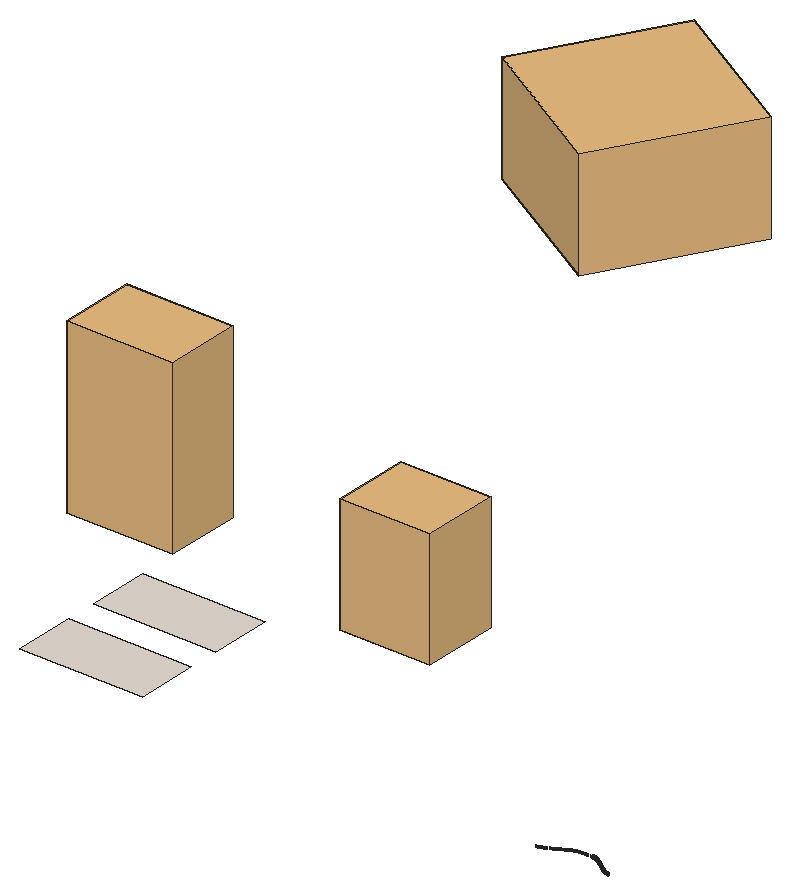
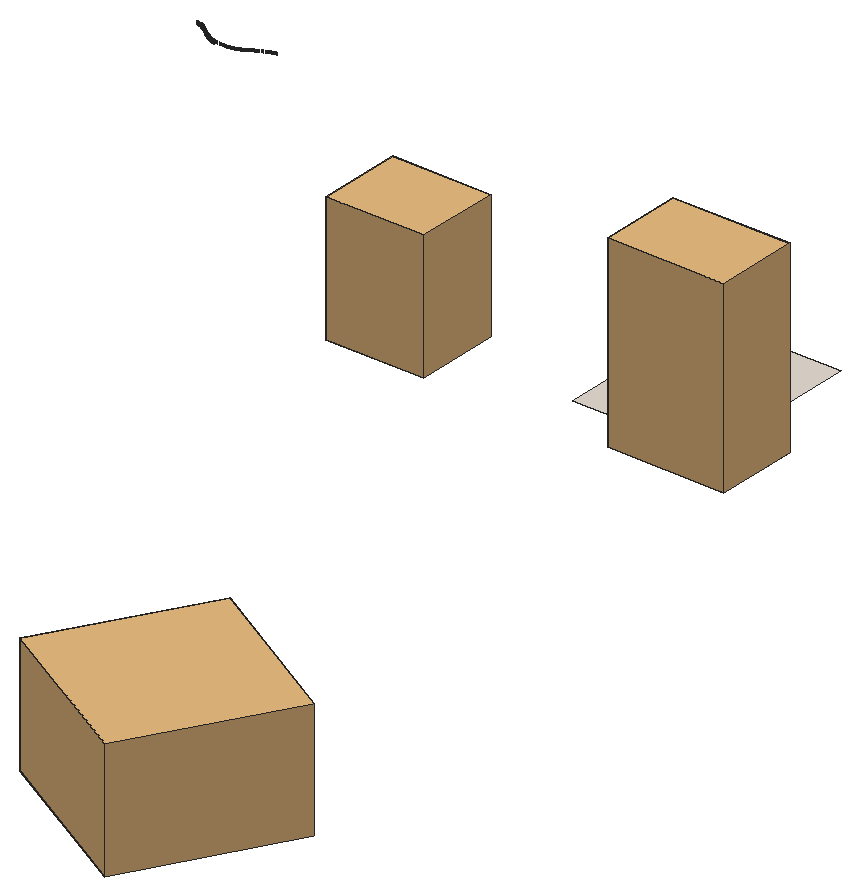
# SketchUp Ruby script. Lengths in inches.
U = 1.inch
M = Sketchup.active_model
def pt(a) = Geom::Point3d.new(a.map { |v| v * U })
def face(e, loops, mat)
  f = e.add_face(loops[0].map { |a| pt(a) })
  loops[1..].each { |l| e.add_face(l.map { |a| pt(a) }).erase! }
  f.material = f.back_material = mat if mat
  f
end
# faces: each face lists its corners as indices into pts; further lists are holes
def faces(e, pts, list, mat = nil) = list.each { |f| face(e, (f[0].is_a?(Array) ? f : [f]).map { |l| l.map { |i| pts[i] } }, mat) }
# xy, xz, yz: faces in a plane at the given z, y or x. An outline is a flat list of corners, or four numbers for a rectangle; further outlines are holes
def ring(l) = l.size == 4 ? [[l[0], l[1]], [l[2], l[1]], [l[2], l[3]], [l[0], l[3]]] : l.each_slice(2).to_a
def flat(e, list, mat, &to3) = list.each { |f| face(e, (f[0].is_a?(Array) ? f : [f]).map { |l| ring(l).map { |u, v| to3.(u, v) } }, mat) }
def xy(e, z, list, mat = nil) = flat(e, list, mat) { |x, y| [x, y, z] }
def xz(e, y, list, mat = nil) = flat(e, list, mat) { |x, z| [x, y, z] }
def yz(e, x, list, mat = nil) = flat(e, list, mat) { |y, z| [x, y, z] }
def lines(e, pts, list) = list.each { |a, b| e.add_line(pt(pts[a]), pt(pts[b])) }
# prism: a flat outline (further loops are holes) pulled along v
def prism(e, loops, v, mat = nil)
  f = face(e, loops, mat); d = Geom::Vector3d.new(v.map { |x| x * U })
  f.pushpull(f.normal.samedirection?(d) ? d.length : -d.length)
end
def box(e, o, s, mat = nil) = prism(e, [[o, [o[0] + s[0], o[1], o[2]], [o[0] + s[0], o[1] + s[1], o[2]], [o[0], o[1] + s[1], o[2]]]], [0, 0, s[2]], mat)
def at(x, y, z, deg = 0) = Geom::Transformation.translation(pt([x, y, z])) * Geom::Transformation.rotation(ORIGIN, Z_AXIS, deg.degrees)
def axes(o, x, y, z) = Geom::Transformation.new([*x, 0, *y, 0, *z, 0, *pt(o).to_a, 1])
def part(name) = M.definitions.add(name)
# library, detail: a bought-in or finely detailed component or shape, given as its bounding box
def library(name, o, s) = part(name).tap { |d| box(d.entities, o, s) }
def detail(e, o, s) = box(e.add_group.entities, o, s)
def put(e, d, t, mat = nil) = e.add_instance(d, t).tap { |i| i.material = mat if mat }
def group(e, t, mat = nil) = e.add_group.tap { |g| g.transformation = t; g.material = mat if mat }.entities
root = M.entities
M.materials.add("Marble_01_1K").color = [230, 221, 211]
M.materials.add("Marble_07_1K").color = [36, 34, 36]
c1 = library("Group\#26",[0,0,0],[90.2,76.39,117.66])
c2 = library("Group\#20",[0,0,0],[118.64,83.7,191])
c3 = library("Group\#158",[-18.75,-2.45,9.86],[64.9,62.99,42.73])
xy(root,2,[[111.43,816.64,159.43,840.64],[111.43,852.64,159.43,876.64]],"Marble_01_1K")
xz(root,802.19,[[347.97,18,348,19]],"Marble_07_1K")
xz(root,802.24,[[347.74,18,347.78,19]],"Marble_07_1K")
xz(root,802.27,[[347.58,18,347.62,19]],"Marble_07_1K")
p = [[358.82,796.23,18],[358.7,796.26,18],[358.7,796.26,19],[358.82,796.23,19],[358.47,796.33,18],[358.36,796.36,18],
  [358.36,796.36,19],[358.47,796.33,19],[358.59,796.29,18],[358.59,796.29,19],[358.13,796.4375,18],[358.01,796.48,18],
  [358.01,796.48,19],[358.13,796.4375,19],[358.24,796.4,18],[358.24,796.4,19],[357.9,796.52,18],[357.79,796.5625,18],
  [357.79,796.5625,19],[357.9,796.52,19],[357.5625,796.65,18],[357.45,796.69,18],[357.45,796.69,19],[357.5625,796.65,19],
  [357.68,796.6,18],[357.68,796.6,19],[357.34,796.74,18],[357.23,796.79,18],[357.23,796.79,19],[357.34,796.74,19],
  [357.12,796.84,18],[357.01,796.89,18],[357.01,796.89,19],[357.12,796.84,19],[356.9,796.9375,18],[356.79,796.99,18],
  [356.79,796.99,19],[356.9,796.9375,19],[356.68,797.04,18],[356.58,797.1,18],[356.58,797.1,19],[356.68,797.04,19],
  [356.47,797.15,18],[356.47,797.15,19],[356.36,797.21,18],[356.26,797.27,18],[356.26,797.27,19],[356.36,797.21,19],
  [356.15,797.32,18],[356.05,797.38,18],[356.05,797.38,19],[356.15,797.32,19],[355.94,797.44,18],[355.84,797.51,18],
  [355.84,797.51,19],[355.94,797.44,19],[355.74,797.57,18],[355.74,797.57,19],[355.64,797.63,18],[355.53,797.7,18],
  [355.53,797.7,19],[355.64,797.63,19],[355.43,797.76,18],[355.43,797.76,19],[355.33,797.83,18],[355.23,797.9,18],
  [355.23,797.9,19],[355.33,797.83,19],[355.13,797.97,18],[355.13,797.97,19],[355.04,798.04,18],[354.9375,798.11,18],
  [354.9375,798.11,19],[355.04,798.04,19],[354.84,798.18,18],[354.84,798.18,19],[354.74,798.25,18],[354.74,798.25,19],
  [354.65,798.33,18],[354.65,798.33,19],[354.55,798.4,18],[354.55,798.4,19],[354.46,798.47,18],[354.46,798.47,19],
  [354.375,798.54,18],[354.29,798.61,18],[354.29,798.61,19],[354.375,798.54,19],[354.2,798.68,18],[354.2,798.68,19],
  [354.11,798.75,18],[354.11,798.75,19],[354.02,798.82,18],[353.93,798.9,18],[353.93,798.9,19],[354.02,798.82,19],
  [353.82,798.99,18],[353.82,798.99,19],[353.71,799.08,18],[353.71,799.08,19],[353.57,799.19,18],[353.57,799.19,19],
  [353.42,799.3,18],[353.42,799.3,19],[353.27,799.42,18],[353.27,799.42,19],[353.14,799.52,18],[353.14,799.52,19],
  [353.02,799.61,18],[353.02,799.61,19],[352.91,799.6875,18],[352.91,799.6875,19],[352.81,799.75,18],[352.81,799.75,19],
  [352.73,799.8125,18],[352.73,799.8125,19],[352.65,799.87,18],[352.65,799.87,19],[352.58,799.92,18],[352.51,799.97,18],
  [352.51,799.97,19],[352.58,799.92,19],[352.45,800.01,18],[352.45,800.01,19],[352.38,800.05,18],[352.38,800.05,19],
  [352.26,800.14,18],[352.21,800.18,18],[352.21,800.18,19],[352.26,800.14,19],[352.32,800.1,18],[352.32,800.1,19],
  [352.15,800.21,18],[352.15,800.21,19],[352.09,800.25,18],[352.09,800.25,19],[351.98,800.33,18],[351.92,800.36,18],
  [351.92,800.36,19],[351.98,800.33,19],[352.04,800.29,18],[352.04,800.29,19],[351.81,800.4375,18],[351.75,800.47,18],
  [351.75,800.47,19],[351.81,800.4375,19],[351.86,800.4,18],[351.86,800.4,19],[351.69,800.51,18],[351.63,800.54,18],
  [351.63,800.54,19],[351.69,800.51,19],[351.58,800.58,18],[351.58,800.58,19],[351.52,800.62,18],[351.52,800.62,19],
  [351.46,800.65,18],[351.46,800.65,19],[351.4,800.6875,18],[351.34,800.72,18],[351.34,800.72,19],[351.4,800.6875,19],
  [351.29,800.76,18],[351.29,800.76,19],[351.17,800.83,18],[351.11,800.86,18],[351.11,800.86,19],[351.17,800.83,19],
  [351.23,800.79,18],[351.23,800.79,19],[350.99,800.93,18],[350.93,800.96,18],[350.93,800.96,19],[350.99,800.93,19],
  [351.05,800.9,18],[351.05,800.9,19],[350.875,801,18],[350.82,801.03,18],[350.82,801.03,19],[350.875,801,19],
  [350.76,801.06,18],[350.76,801.06,19],[350.7,801.1,18],[350.64,801.13,18],[350.64,801.13,19],[350.7,801.1,19],
  [350.58,801.16,18],[350.58,801.16,19],[350.46,801.23,18],[350.41,801.26,18],[350.41,801.26,19],[350.46,801.23,19],
  [350.52,801.2,18],[350.52,801.2,19],[350.25,801.34,18],[350.21,801.36,18],[350.21,801.36,19],[350.25,801.34,19],
  [350.35,801.29,18],[350.3,801.3125,18],[350.3,801.3125,19],[350.35,801.29,19],[350.08,801.43,18],[350.05,801.45,18],
  [350.05,801.45,19],[350.08,801.43,19],[350.01,801.46,18],[350.01,801.46,19],[350.16,801.39,18],[350.12,801.41,18],
  [350.12,801.41,19],[350.16,801.39,19],[349.87,801.53,18],[349.83,801.55,18],[349.83,801.55,19],[349.87,801.53,19],
  [349.8,801.56,18],[349.8,801.56,19],[349.97,801.48,18],[349.94,801.5,18],[349.94,801.5,19],[349.97,801.48,19],
  [349.91,801.51,18],[349.91,801.51,19],[349.66,801.63,18],[349.62,801.64,18],[349.62,801.64,19],[349.66,801.63,19],
  [349.59,801.66,18],[349.59,801.66,19],[349.76,801.58,18],[349.73,801.6,18],[349.73,801.6,19],[349.76,801.58,19],
  [349.69,801.61,18],[349.69,801.61,19],[349.39,801.74,18],[349.35,801.76,18],[349.35,801.76,19],[349.39,801.74,19],
  [349.47,801.71,18],[349.43,801.72,18],[349.43,801.72,19],[349.47,801.71,19],[349.55,801.68,18],[349.51,801.69,18],
  [349.51,801.69,19],[349.55,801.68,19],[349.2,801.82,18],[349.13,801.84,18],[349.13,801.84,19],[349.2,801.82,19],
  [349.0625,801.87,18],[349.0625,801.87,19],[349.25,801.8,18],[349.25,801.8,19],[349.3,801.78,18],[349.3,801.78,19],
  [348.89,801.93,18],[348.79,801.97,18],[348.79,801.97,19],[348.89,801.93,19],[348.98,801.9,18],[348.98,801.9,19],
  [348.59,802.03,18],[348.51,802.05,18],[348.51,802.05,19],[348.59,802.03,19],[348.68,802,18],[348.68,802,19],
  [348.17,802.14,18],[348.125,802.16,18],[348.125,802.16,19],[348.17,802.14,19],[348.26,802.12,18],[348.22,802.13,18],
  [348.22,802.13,19],[348.26,802.12,19],[348.375,802.09,18],[348.32,802.11,18],[348.32,802.11,19],[348.375,802.09,19],
  [348.4375,802.07,18],[348.4375,802.07,19],[347.74,802.24,18],[347.7,802.25,18],[347.7,802.25,19],[347.74,802.24,19],
  [347.85,802.22,18],[347.8125,802.23,18],[347.8125,802.23,19],[347.85,802.22,19],[347.78,802.24,18],[347.78,802.24,19],
  [347.97,802.19,18],[347.93,802.2,18],[347.93,802.2,19],[347.97,802.19,19],[347.89,802.21,18],[347.89,802.21,19],
  [348.08,802.17,18],[348.04,802.18,18],[348.04,802.18,19],[348.08,802.17,19],[348,802.19,18],[348,802.19,19],
  [347.58,802.27,18],[347.55,802.28,18],[347.55,802.28,19],[347.58,802.27,19],[347.51,802.29,18],[347.51,802.29,19],
  [347.47,802.3,18],[347.47,802.3,19],[347.66,802.26,18],[347.62,802.27,18],[347.62,802.27,19],[347.66,802.26,19],
  [346.2,801.84,18],[346.2,801.84,19],[346.86,801.77,18],[346.86,801.77,19],[346.0625,801.85,18],[346.0625,801.85,19],
  [345.91,801.86,18],[345.91,801.86,19],[345.75,801.87,18],[345.75,801.87,19],[345.59,801.88,18],[345.59,801.88,19],
  [345.41,801.89,18],[345.41,801.89,19],[345.23,801.9,18],[345.23,801.9,19],[345.04,801.91,18],[345.04,801.91,19],
  [344.85,801.91,18],[344.85,801.91,19],[344.66,801.92,18],[344.66,801.92,19],[344.47,801.92,18],[344.47,801.92,19],
  [344.29,801.92,18],[344.29,801.92,19],[344.1,801.92,18],[344.1,801.92,19],[343.93,801.91,18],[343.93,801.91,19],
  [343.77,801.91,18],[343.77,801.91,19],[343.61,801.9,18],[343.61,801.9,19],[343.47,801.89,18],[343.47,801.89,19],
  [343.34,801.875,18],[343.34,801.875,19],[343.21,801.86,18],[343.21,801.86,19],[343.09,801.84,18],[343.09,801.84,19],
  [342.97,801.83,18],[342.97,801.83,19],[342.85,801.81,18],[342.85,801.81,19],[342.74,801.79,18],[342.74,801.79,19],
  [342.625,801.77,18],[342.625,801.77,19],[342.51,801.75,18],[342.51,801.75,19],[342.4,801.72,18],[342.4,801.72,19],
  [342.29,801.7,18],[342.29,801.7,19],[342.17,801.68,18],[342.17,801.68,19],[342.0625,801.65,18],[342.0625,801.65,19],
  [341.95,801.63,18],[341.95,801.63,19],[341.84,801.6,18],[341.84,801.6,19],[341.72,801.57,18],[341.72,801.57,19],
  [341.61,801.55,18],[341.61,801.55,19],[341.51,801.52,18],[341.51,801.52,19],[341.4,801.49,18],[341.4,801.49,19],
  [341.3,801.47,18],[341.3,801.47,19],[341.21,801.44,18],[341.21,801.44,19],[341.125,801.42,18],[341.125,801.42,19],
  [341.05,801.4,18],[341.05,801.4,19],[340.98,801.38,18],[340.98,801.38,19],[340.92,801.36,18],[340.92,801.36,19],
  [340.875,801.35,18],[340.875,801.35,19],[340.83,801.34,18],[340.83,801.34,19],[340.79,801.32,18],[340.79,801.32,19],
  [340.75,801.3125,18],[340.75,801.3125,19],[340.72,801.3,18],[340.72,801.3,19],[340.6875,801.29,18],[340.6875,801.29,19],
  [340.66,801.28,18],[340.66,801.28,19],[340.625,801.27,18],[340.625,801.27,19],[340.59,801.26,18],[340.59,801.26,19],
  [340.5625,801.25,18],[340.5625,801.25,19],[340.53,801.24,18],[340.53,801.24,19],[340.5,801.23,18],[340.5,801.23,19],
  [340.47,801.22,18],[340.47,801.22,19],[340.44,801.21,18],[340.44,801.21,19],[340.4,801.19,18],[340.4,801.19,19],
  [340.37,801.18,18],[340.37,801.18,19],[340.34,801.17,18],[340.34,801.17,19],[340.31,801.16,18],[340.31,801.16,19],
  [340.28,801.15,18],[340.28,801.15,19],[340.25,801.14,18],[340.25,801.14,19],[340.22,801.125,18],[340.22,801.125,19],
  [340.18,801.11,18],[340.18,801.11,19],[340.15,801.1,18],[340.15,801.1,19],[340.12,801.09,18],[340.12,801.09,19],
  [340.09,801.08,18],[340.09,801.08,19],[340.06,801.0625,18],[340.06,801.0625,19],[340.02,801.05,18],[340.02,801.05,19],
  [339.99,801.04,18],[339.99,801.04,19],[339.95,801.02,18],[339.95,801.02,19],[339.92,801.01,18],[339.92,801.01,19],
  [339.875,800.99,18],[339.875,800.99,19],[339.83,800.97,18],[339.83,800.97,19],[339.79,800.95,18],[339.79,800.95,19],
  [339.73,800.93,18],[339.73,800.93,19],[339.67,800.9,18],[339.67,800.9,19],[339.61,800.87,18],[339.61,800.87,19],
  [339.53,800.84,18],[339.53,800.84,19],[339.45,800.8,18],[339.45,800.8,19],[339.36,800.76,18],[339.36,800.76,19],
  [339.29,800.72,18],[339.29,800.72,19],[339.22,800.6875,18],[339.22,800.6875,19],[339.16,800.66,18],[339.16,800.66,19],
  [339.11,800.63,18],[339.11,800.63,19],[339.07,800.61,18],[339.07,800.61,19],[339.03,800.59,18],[339.03,800.59,19],
  [338.99,800.57,18],[338.99,800.57,19],[338.95,800.55,18],[338.95,800.55,19],[338.92,800.53,18],[338.92,800.53,19],
  [338.89,800.51,18],[338.89,800.51,19],[338.85,800.49,18],[338.85,800.49,19],[338.82,800.48,18],[338.82,800.48,19],
  [338.79,800.46,18],[338.79,800.46,19],[338.76,800.44,18],[338.76,800.44,19],[338.73,800.43,18],[338.73,800.43,19],
  [338.71,800.41,18],[338.71,800.41,19],[338.68,800.39,18],[338.68,800.39,19],[338.65,800.375,18],[338.65,800.375,19],
  [338.62,800.36,18],[338.62,800.36,19],[338.59,800.34,18],[338.59,800.34,19],[338.5625,800.32,18],[338.5625,800.32,19],
  [338.53,800.31,18],[338.53,800.31,19],[338.5,800.29,18],[338.5,800.29,19],[338.48,800.27,18],[338.48,800.27,19],
  [338.45,800.25,18],[338.45,800.25,19],[338.42,800.24,18],[338.42,800.24,19],[338.39,800.22,18],[338.39,800.22,19],
  [338.36,800.2,18],[338.36,800.2,19],[338.33,800.18,18],[338.33,800.18,19],[338.31,800.17,18],[338.31,800.17,19],
  [338.28,800.15,18],[338.28,800.15,19],[338.25,800.13,18],[338.25,800.13,19],[338.22,800.11,18],[338.22,800.11,19],
  [338.18,800.09,18],[338.18,800.09,19],[338.14,800.0625,18],[338.14,800.0625,19],[338.1,800.03,18],[338.1,800.03,19],
  [338.04,800,18],[338.04,800,19],[337.97,799.96,18],[337.97,799.96,19],[337.89,799.91,18],[337.89,799.91,19],
  [337.8,799.85,18],[337.8,799.85,19],[337.6875,799.79,18],[337.6875,799.79,19],[337.57,799.72,18],[337.57,799.72,19],
  [337.44,799.64,18],[337.44,799.64,19],[337.3,799.56,18],[337.3,799.56,19],[337.16,799.48,18],[337.16,799.48,19],
  [337.01,799.39,18],[337.01,799.39,19],[336.86,799.3,18],[336.86,799.3,19],[336.71,799.22,18],[336.71,799.22,19],
  [336.5625,799.13,18],[336.5625,799.13,19],[336.41,799.05,18],[336.41,799.05,19],[336.25,798.96,18],[336.25,798.96,19],
  [336.09,798.875,18],[336.09,798.875,19],[335.92,798.78,18],[335.92,798.78,19],[335.74,798.69,18],[335.74,798.69,19],
  [335.55,798.59,18],[335.55,798.59,19],[335.36,798.49,18],[335.36,798.49,19],[335.14,798.38,18],[335.14,798.38,19],
  [334.91,798.27,18],[334.91,798.27,19],[334.64,798.14,18],[334.64,798.14,19],[334.34,797.99,18],[334.34,797.99,19],
  [334,797.83,18],[334,797.83,19],[333.61,797.65,18],[333.61,797.65,19],[333.17,797.45,18],[333.17,797.45,19],
  [332.96,797.34,18],[332.96,797.34,19],[332.76,797.25,18],[332.76,797.25,19],[332.59,797.17,18],[332.59,797.17,19],
  [332.44,797.1,18],[332.44,797.1,19],[332.31,797.04,18],[332.31,797.04,19],[332.1875,796.99,18],[332.1875,796.99,19],
  [332.08,796.95,18],[332.08,796.95,19],[331.98,796.9,18],[331.98,796.9,19],[331.88,796.87,18],[331.88,796.87,19],
  [331.79,796.83,18],[331.79,796.83,19],[331.7,796.79,18],[331.7,796.79,19],[331.61,796.76,18],[331.61,796.76,19],
  [331.53,796.73,18],[331.53,796.73,19],[331.44,796.7,18],[331.44,796.7,19],[331.36,796.67,18],[331.36,796.67,19],
  [331.28,796.64,18],[331.28,796.64,19],[331.2,796.61,18],[331.2,796.61,19],[331.12,796.59,18],[331.12,796.59,19],
  [331.04,796.56,18],[331.04,796.56,19],[330.95,796.53,18],[330.95,796.53,19],[330.875,796.51,18],[330.875,796.51,19],
  [330.79,796.48,18],[330.79,796.48,19],[330.71,796.46,18],[330.71,796.46,19],[330.625,796.43,18],[330.625,796.43,19],
  [330.54,796.41,18],[330.54,796.41,19],[330.46,796.39,18],[330.46,796.39,19],[330.38,796.36,18],[330.38,796.36,19],
  [330.3,796.34,18],[330.3,796.34,19],[330.21,796.32,18],[330.21,796.32,19],[330.13,796.3,18],[330.13,796.3,19],
  [330.05,796.28,18],[330.05,796.28,19],[329.96,796.26,18],[329.96,796.26,19],[329.88,796.24,18],[329.88,796.24,19],
  [356.99,796.23,18],[356.99,796.23,19],[356.875,796.29,18],[356.875,796.29,19],[356.76,796.34,18],[356.76,796.34,19],
  [356.64,796.39,18],[356.64,796.39,19],[356.53,796.45,18],[356.53,796.45,19],[356.42,796.5,18],[356.42,796.5,19],
  [356.3,796.56,18],[356.3,796.56,19],[356.19,796.62,18],[356.19,796.62,19],[356.08,796.68,18],[356.08,796.68,19],
  [355.97,796.74,18],[355.97,796.74,19],[355.86,796.8,18],[355.86,796.8,19],[355.75,796.86,18],[355.75,796.86,19],
  [355.64,796.92,18],[355.64,796.92,19],[355.53,796.99,18],[355.53,796.99,19],[355.42,797.05,18],[355.42,797.05,19],
  [355.3125,797.12,18],[355.3125,797.12,19],[355.21,797.19,18],[355.21,797.19,19],[355.1,797.26,18],[355.1,797.26,19],
  [355,797.33,18],[355,797.33,19],[354.89,797.4,18],[354.89,797.4,19],[354.79,797.47,18],[354.79,797.47,19],
  [354.69,797.55,18],[354.69,797.55,19],[354.58,797.62,18],[354.58,797.62,19],[354.48,797.69,18],[354.48,797.69,19],
  [354.38,797.77,18],[354.38,797.77,19],[354.29,797.84,18],[354.29,797.84,19],[354.2,797.91,18],[354.2,797.91,19],
  [354.11,797.98,18],[354.11,797.98,19],[354.02,798.05,18],[354.02,798.05,19],[353.94,798.11,18],[353.94,798.11,19],
  [353.87,798.17,18],[353.87,798.17,19],[353.81,798.22,18],[353.81,798.22,19],[353.74,798.27,18],[353.74,798.27,19],
  [353.68,798.32,18],[353.68,798.32,19],[353.63,798.37,18],[353.63,798.37,19],[353.57,798.41,18],[353.57,798.41,19],
  [353.52,798.45,18],[353.52,798.45,19],[353.47,798.5,18],[353.47,798.5,19],[353.42,798.54,18],[353.42,798.54,19],
  [353.37,798.58,18],[353.37,798.58,19],[353.32,798.62,18],[353.32,798.62,19],[353.26,798.66,18],[353.26,798.66,19],
  [353.21,798.7,18],[353.21,798.7,19],[353.16,798.74,18],[353.16,798.74,19],[353.11,798.78,18],[353.11,798.78,19],
  [353.06,798.82,18],[353.06,798.82,19],[353,798.86,18],[353,798.86,19],[352.95,798.9,18],[352.95,798.9,19],
  [352.9,798.94,18],[352.9,798.94,19],[352.84,798.98,18],[352.84,798.98,19],[352.79,799.02,18],[352.79,799.02,19],
  [352.74,799.0625,18],[352.74,799.0625,19],[352.68,799.1,18],[352.68,799.1,19],[352.63,799.14,18],[352.63,799.14,19],
  [352.58,799.18,18],[352.58,799.18,19],[352.52,799.22,18],[352.52,799.22,19],[352.47,799.26,18],[352.47,799.26,19],
  [352.42,799.3,18],[352.42,799.3,19],[352.36,799.34,18],[352.36,799.34,19],[352.31,799.375,18],[352.31,799.375,19],
  [352.25,799.41,18],[352.25,799.41,19],[352.2,799.45,18],[352.2,799.45,19],[352.15,799.49,18],[352.15,799.49,19],
  [352.09,799.52,18],[352.09,799.52,19],[352.04,799.5625,18],[352.04,799.5625,19],[351.98,799.6,18],[351.98,799.6,19],
  [351.93,799.64,18],[351.93,799.64,19],[351.87,799.67,18],[351.87,799.67,19],[351.82,799.71,18],[351.82,799.71,19],
  [351.76,799.75,18],[351.76,799.75,19],[351.71,799.78,18],[351.71,799.78,19],[351.65,799.82,18],[351.65,799.82,19],
  [351.59,799.85,18],[351.59,799.85,19],[351.54,799.89,18],[351.54,799.89,19],[351.48,799.93,18],[351.48,799.93,19],
  [351.43,799.96,18],[351.43,799.96,19],[351.37,800,18],[351.37,800,19],[351.31,800.03,18],[351.31,800.03,19],
  [351.26,800.07,18],[351.26,800.07,19],[351.2,800.1,18],[351.2,800.1,19],[351.15,800.14,18],[351.15,800.14,19],
  [351.09,800.17,18],[351.09,800.17,19],[351.03,800.21,18],[351.03,800.21,19],[350.98,800.24,18],[350.98,800.24,19],
  [350.92,800.27,18],[350.92,800.27,19],[350.86,800.31,18],[350.86,800.31,19],[350.8,800.34,18],[350.8,800.34,19],
  [350.75,800.375,18],[350.75,800.375,19],[350.69,800.41,18],[350.69,800.41,19],[350.63,800.44,18],[350.63,800.44,19],
  [350.58,800.47,18],[350.58,800.47,19],[350.52,800.51,18],[350.52,800.51,19],[350.46,800.54,18],[350.46,800.54,19],
  [350.4,800.57,18],[350.4,800.57,19],[350.34,800.6,18],[350.34,800.6,19],[350.29,800.63,18],[350.29,800.63,19],
  [350.23,800.67,18],[350.23,800.67,19],[350.17,800.7,18],[350.17,800.7,19],[350.12,800.73,18],[350.12,800.73,19],
  [350.07,800.75,18],[350.07,800.75,19],[350.02,800.78,18],[350.02,800.78,19],[349.97,800.8,18],[349.97,800.8,19],
  [349.93,800.83,18],[349.93,800.83,19],[349.89,800.85,18],[349.89,800.85,19],[349.85,800.87,18],[349.85,800.87,19],
  [349.8125,800.89,18],[349.8125,800.89,19],[349.78,800.91,18],[349.78,800.91,19],[349.74,800.92,18],[349.74,800.92,19],
  [349.71,800.9375,18],[349.71,800.9375,19],[349.68,800.95,18],[349.68,800.95,19],[349.64,800.97,18],[349.64,800.97,19],
  [349.61,800.99,18],[349.61,800.99,19],[349.58,801,18],[349.58,801,19],[349.55,801.02,18],[349.55,801.02,19],
  [349.51,801.03,18],[349.51,801.03,19],[349.48,801.05,18],[349.48,801.05,19],[349.45,801.0625,18],[349.45,801.0625,19],
  [349.41,801.08,18],[349.41,801.08,19],[349.38,801.09,18],[349.38,801.09,19],[349.35,801.11,18],[349.35,801.11,19],
  [349.3125,801.12,18],[349.3125,801.12,19],[349.28,801.14,18],[349.28,801.14,19],[349.25,801.15,18],[349.25,801.15,19],
  [349.21,801.16,18],[349.21,801.16,19],[349.18,801.18,18],[349.18,801.18,19],[349.15,801.19,18],[349.15,801.19,19],
  [349.11,801.2,18],[349.11,801.2,19],[349.08,801.22,18],[349.08,801.22,19],[349.04,801.23,18],[349.04,801.23,19],
  [349.01,801.24,18],[349.01,801.24,19],[348.98,801.26,18],[348.98,801.26,19],[348.94,801.27,18],[348.94,801.27,19],
  [348.91,801.28,18],[348.91,801.28,19],[348.875,801.3,18],[348.875,801.3,19],[348.84,801.31,18],[348.84,801.31,19],
  [348.81,801.32,18],[348.81,801.32,19],[348.77,801.33,18],[348.77,801.33,19],[348.74,801.34,18],[348.74,801.34,19],
  [348.7,801.36,18],[348.7,801.36,19],[348.67,801.37,18],[348.67,801.37,19],[348.63,801.38,18],[348.63,801.38,19],
  [348.6,801.39,18],[348.6,801.39,19],[348.56,801.4,18],[348.56,801.4,19],[348.53,801.41,18],[348.53,801.41,19],
  [348.5,801.42,18],[348.5,801.42,19],[348.46,801.44,18],[348.46,801.44,19],[348.43,801.45,18],[348.43,801.45,19],
  [348.39,801.46,18],[348.39,801.46,19],[348.36,801.47,18],[348.36,801.47,19],[348.32,801.48,18],[348.32,801.48,19],
  [348.29,801.49,18],[348.29,801.49,19],[348.25,801.5,18],[348.25,801.5,19],[348.22,801.51,18],[348.22,801.51,19],
  [348.18,801.52,18],[348.18,801.52,19],[348.15,801.53,18],[348.15,801.53,19],[348.11,801.54,18],[348.11,801.54,19],
  [348.08,801.55,18],[348.08,801.55,19],[348.04,801.55,18],[348.04,801.55,19],[348.01,801.5625,18],[348.01,801.5625,19],
  [347.97,801.57,18],[347.97,801.57,19],[347.94,801.58,18],[347.94,801.58,19],[347.9,801.59,18],[347.9,801.59,19],
  [347.86,801.6,18],[347.86,801.6,19],[347.83,801.61,18],[347.83,801.61,19],[347.79,801.61,18],[347.79,801.61,19],
  [347.76,801.62,18],[347.76,801.62,19],[347.72,801.63,18],[347.72,801.63,19],[347.6875,801.64,18],[347.6875,801.64,19],
  [347.65,801.65,18],[347.65,801.65,19],[347.62,801.65,18],[347.62,801.65,19],[347.58,801.66,18],[347.58,801.66,19],
  [347.54,801.67,18],[347.54,801.67,19],[347.51,801.67,18],[347.51,801.67,19],[347.47,801.68,18],[347.47,801.68,19],
  [347.4375,801.6875,18],[347.4375,801.6875,19],[347.4,801.69,18],[347.4,801.69,19],[347.37,801.7,18],[347.37,801.7,19],
  [347.33,801.71,18],[347.33,801.71,19],[347.29,801.71,18],[347.29,801.71,19],[347.26,801.72,18],[347.26,801.72,19],
  [347.22,801.72,18],[347.22,801.72,19],[347.1875,801.73,18],[347.1875,801.73,19],[347.15,801.74,18],[347.15,801.74,19],
  [347.11,801.74,18],[347.11,801.74,19],[347.08,801.75,18],[347.08,801.75,19],[347.04,801.75,18],[347.04,801.75,19],
  [347.01,801.76,18],[347.01,801.76,19],[346.97,801.76,18],[346.97,801.76,19],[346.93,801.77,18],[346.93,801.77,19],
  [346.9,801.77,18],[346.9,801.77,19]]
faces(root,p,[[0,1,2,3],[4,5,6,7],[8,4,7,9],[1,8,9,2],[10,11,12,13],[14,10,13,15],[5,14,15,6],[16,17,18,19],
  [11,16,19,12],[20,21,22,23],[24,20,23,25],[17,24,25,18],[26,27,28,29],[21,26,29,22],[30,31,32,33],[27,30,33,28],
  [34,35,36,37],[31,34,37,32],[38,39,40,41],[35,38,41,36],[39,42,43,40],[44,45,46,47],[42,44,47,43],[48,49,50,51],
  [45,48,51,46],[52,53,54,55],[49,52,55,50],[53,56,57,54],[58,59,60,61],[56,58,61,57],[59,62,63,60],[64,65,66,67],
  [62,64,67,63],[65,68,69,66],[70,71,72,73],[68,70,73,69],[71,74,75,72],[74,76,77,75],[76,78,79,77],[78,80,81,79],
  [80,82,83,81],[84,85,86,87],[82,84,87,83],[85,88,89,86],[88,90,91,89],[92,93,94,95],[90,92,95,91],[93,96,97,94],
  [96,98,99,97],[98,100,101,99],[100,102,103,101],[102,104,105,103],[104,106,107,105],[106,108,109,107],[108,110,111,109],[110,112,113,111],
  [112,114,115,113],[114,116,117,115],[118,119,120,121],[116,118,121,117],[119,122,123,120],[122,124,125,123],[126,127,128,129],[124,130,131,125],
  [130,126,129,131],[127,132,133,128],[132,134,135,133],[136,137,138,139],[134,140,141,135],[140,136,139,141],[142,143,144,145],[146,142,145,147],
  [137,146,147,138],[148,149,150,151],[149,152,153,150],[143,148,151,144],[152,154,155,153],[154,156,157,155],[158,159,160,161],[159,162,163,160],
  [156,158,161,157],[164,165,166,167],[162,168,169,163],[168,164,167,169],[170,171,172,173],[174,170,173,175],[165,174,175,166],[176,177,178,179],
  [177,180,181,178],[171,176,179,172],[182,183,184,185],[183,186,187,184],[180,182,185,181],[188,189,190,191],[186,192,193,187],[192,188,191,193],
  [194,195,196,197],[198,199,200,201],[199,194,197,200],[189,198,201,190],[202,203,204,205],[203,206,207,204],[208,209,210,211],[209,202,205,210],
  [195,208,211,196],[212,213,214,215],[213,216,217,214],[218,219,220,221],[219,222,223,220],[222,212,215,223],[206,218,221,207],[224,225,226,227],
  [225,228,229,226],[230,231,232,233],[231,234,235,232],[234,224,227,235],[216,230,233,217],[236,237,238,239],[240,241,242,243],[241,236,239,242],
  [244,245,246,247],[245,240,243,246],[228,244,247,229],[248,249,250,251],[249,252,253,250],[254,248,251,255],[237,256,257,238],[256,254,255,257],
  [258,259,260,261],[262,258,261,263],[252,262,263,253],[264,265,266,267],[268,264,267,269],[259,268,269,260],[270,271,272,273],[274,275,276,277],
  [275,270,273,276],[278,279,280,281],[279,274,277,280],[265,282,283,266],[282,278,281,283],[284,285,286,287],[288,289,290,291],[289,292,293,290],
  [294,295,296,297],[295,298,299,296],[298,288,291,299],[300,301,302,303],[301,304,305,302],[271,300,303,272],[306,307,308,309],[307,310,311,308],
  [310,312,313,311],[314,315,316,317],[285,314,317,286]],"Marble_07_1K")
lines(root,p,[[318,319],[320,321],[322,323],[324,325],[326,327],[328,329],[330,331],[332,333],[334,335],[336,337],[338,339],[340,341],
  [342,343],[344,345],[346,347],[348,349],[350,351],[352,353],[354,355],[356,357],[358,359],[360,361],[362,363],[364,365],
  [366,367],[368,369],[370,371],[372,373],[374,375],[376,377],[378,379],[380,381],[382,383],[384,385],[386,387],[388,389],
  [390,391],[392,393],[394,395],[396,397],[398,399],[400,401],[402,403],[404,405],[406,407],[408,409],[410,411],[412,413],
  [414,415],[416,417],[418,419],[420,421],[422,423],[424,425],[426,427],[428,429],[430,431],[432,433],[434,435],[436,437],
  [438,439],[440,441],[442,443],[444,445],[446,447],[448,449],[450,451],[452,453],[454,455],[456,457],[458,459],[460,461],
  [462,463],[464,465],[466,467],[468,469],[470,471],[472,473],[474,475],[476,477],[478,479],[480,481],[482,483],[484,485],
  [486,487],[488,489],[490,491],[492,493],[494,495],[496,497],[498,499],[500,501],[502,503],[504,505],[506,507],[508,509],
  [510,511],[512,513],[514,515],[516,517],[518,519],[520,521],[522,523],[524,525],[526,527],[528,529],[530,531],[532,533],
  [534,535],[536,537],[538,539],[540,541],[542,543],[544,545],[546,547],[548,549],[550,551],[552,553],[554,555],[556,557],
  [558,559],[560,561],[562,563],[564,565],[566,567],[568,569],[570,571],[572,573],[574,575],[576,577],[578,579],[580,581],
  [582,583],[584,585],[586,587],[588,589],[590,591],[592,593],[594,595],[596,597],[598,599],[600,601],[602,603],[604,605],
  [606,607],[608,609],[610,611],[612,613],[614,615],[616,617],[618,619],[620,621],[622,623],[624,625],[626,627],[628,629],
  [630,631],[632,633],[634,635],[636,637],[638,639],[640,641],[642,643],[644,645],[646,647],[648,649],[650,651],[652,653],
  [654,655],[656,657],[658,659],[660,661],[662,663],[664,665],[666,667],[668,669],[670,671],[672,673],[674,675],[676,677],
  [678,679],[680,681],[682,683],[684,685],[686,687],[688,689],[690,691],[692,693],[694,695],[696,697],[698,699],[700,701],
  [702,703],[704,705],[706,707],[708,709],[710,711],[712,713],[714,715],[716,717],[718,719],[720,721],[722,723],[724,725],
  [726,727],[728,729],[730,731],[732,733],[734,735],[736,737],[738,739],[740,741],[742,743],[744,745],[746,747],[748,749],
  [750,751],[752,753],[754,755],[756,757],[758,759],[760,761],[762,763],[764,765],[766,767],[768,769],[770,771],[772,773],
  [774,775],[776,777],[778,779],[780,781],[782,783],[784,785],[786,787],[788,789],[790,791],[792,793],[794,795],[796,797],
  [798,799],[800,801],[802,803],[804,805],[806,807],[808,809],[810,811],[812,813],[814,815],[816,817],[818,819],[820,821],
  [822,823],[824,825],[826,827],[828,829],[830,831],[832,833],[834,835],[836,837],[838,839],[840,841],[842,843],[844,845],
  [846,847],[848,849],[850,851],[852,853],[854,855],[856,857],[858,859],[860,861],[862,863],[864,865],[866,867],[868,869],
  [870,871],[872,873],[874,875],[876,877],[878,879],[880,881],[882,883],[884,885],[886,887],[888,889],[890,891],[892,893],
  [894,895],[896,897],[898,899],[900,901],[902,903],[904,905],[906,907],[908,909],[910,911],[912,913],[914,915],[916,917],
  [918,919],[920,921],[922,923],[924,925],[926,927],[928,929],[930,931],[932,933],[934,935],[936,937],[938,939],[940,941],
  [942,943],[944,945],[946,947],[948,949],[950,951],[952,953],[954,955],[956,957],[958,959],[960,961],[962,963],[964,965],
  [966,967],[968,969],[970,971],[972,973],[974,975],[976,977],[978,979],[980,981],[982,983],[984,985],[986,987],[988,989],
  [990,991],[992,993],[994,995],[996,997],[998,999],[1000,1001],[1002,1003],[1004,1005],[1006,1007],[1008,1009],[1010,1011],[1012,1013],
  [1014,1015],[1016,1017],[1018,1019],[1020,1021],[1022,1023],[1024,1025],[1026,1027],[1028,1029],[1030,1031],[1032,1033],[1034,1035],[1036,1037],
  [1038,1039],[1040,1041],[1042,1043],[1044,1045],[1046,1047],[1048,1049],[1050,1051]])
put(root,c1,axes([190.34,875.01,10.88],[0.39,0,0],[0,0.39,0],[0,0,0.39]))
put(root,c2,axes([81.5,876.97,12.93],[0.352,0,0],[0,0.352,0],[0,0,0.352]))
put(root,c3,at(69.31,1120.125,0,-30))
